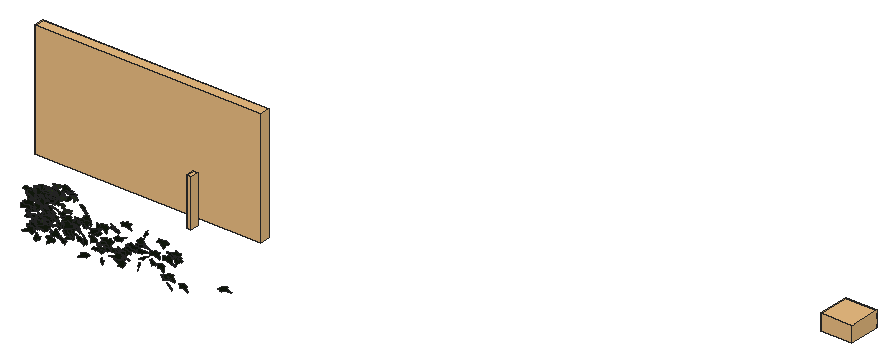
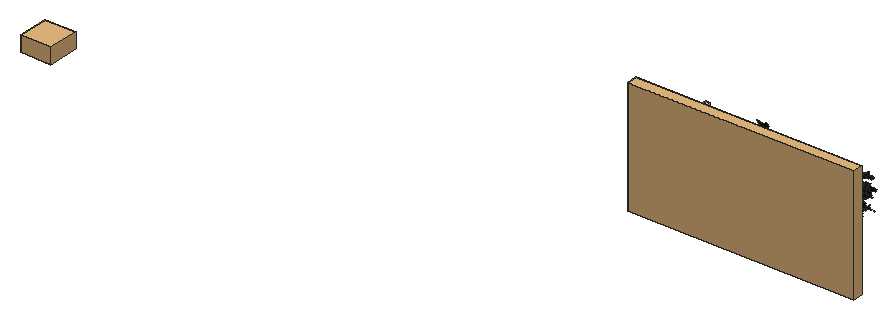
# SketchUp Ruby script. Lengths in millimetres.
U = 1.mm
M = Sketchup.active_model
def pt(a) = Geom::Point3d.new(a.map { |v| v * U })
def face(e, loops, mat)
  f = e.add_face(loops[0].map { |a| pt(a) })
  loops[1..].each { |l| e.add_face(l.map { |a| pt(a) }).erase! }
  f.material = f.back_material = mat if mat
  f
end
# faces: each face lists its corners as indices into pts; further lists are holes
def faces(e, pts, list, mat = nil) = list.each { |f| face(e, (f[0].is_a?(Array) ? f : [f]).map { |l| l.map { |i| pts[i] } }, mat) }
# xy, xz, yz: faces in a plane at the given z, y or x. An outline is a flat list of corners, or four numbers for a rectangle; further outlines are holes
def ring(l) = l.size == 4 ? [[l[0], l[1]], [l[2], l[1]], [l[2], l[3]], [l[0], l[3]]] : l.each_slice(2).to_a
def flat(e, list, mat, &to3) = list.each { |f| face(e, (f[0].is_a?(Array) ? f : [f]).map { |l| ring(l).map { |u, v| to3.(u, v) } }, mat) }
def xy(e, z, list, mat = nil) = flat(e, list, mat) { |x, y| [x, y, z] }
def xz(e, y, list, mat = nil) = flat(e, list, mat) { |x, z| [x, y, z] }
def yz(e, x, list, mat = nil) = flat(e, list, mat) { |y, z| [x, y, z] }
def lines(e, pts, list) = list.each { |a, b| e.add_line(pt(pts[a]), pt(pts[b])) }
# prism: a flat outline (further loops are holes) pulled along v
def prism(e, loops, v, mat = nil)
  f = face(e, loops, mat); d = Geom::Vector3d.new(v.map { |x| x * U })
  f.pushpull(f.normal.samedirection?(d) ? d.length : -d.length)
end
def box(e, o, s, mat = nil) = prism(e, [[o, [o[0] + s[0], o[1], o[2]], [o[0] + s[0], o[1] + s[1], o[2]], [o[0], o[1] + s[1], o[2]]]], [0, 0, s[2]], mat)
def at(x, y, z, deg = 0) = Geom::Transformation.translation(pt([x, y, z])) * Geom::Transformation.rotation(ORIGIN, Z_AXIS, deg.degrees)
def axes(o, x, y, z) = Geom::Transformation.new([*x, 0, *y, 0, *z, 0, *pt(o).to_a, 1])
def part(name) = M.definitions.add(name)
# library, detail: a bought-in or finely detailed component or shape, given as its bounding box
def library(name, o, s) = part(name).tap { |d| box(d.entities, o, s) }
def detail(e, o, s) = box(e.add_group.entities, o, s)
def put(e, d, t, mat = nil) = e.add_instance(d, t).tap { |i| i.material = mat if mat }
def group(e, t, mat = nil) = e.add_group.tap { |g| g.transformation = t; g.material = mat if mat }.entities
root = M.entities
M.materials.add("efeu1").color = [18, 25, 13]
M.materials.add("efeu2").color = [43, 57, 29]
c1 = part("ivyleaf_9")
p = [[39.1,54.8,31.7],[34.5,51.8,30.2],[-5.3,25.2,17.3],[-17.9,28.3,20.9],[-21.6,21.7,17],[-20.2,4.3,5.3],
  [-22.9,-0.3,2.5],[-17.1,-4,-0.6],[-2,-2.1,-1.2],[-0.7,-15.4,-10.1],[16.6,-22.3,-16.7],[21.1,-15.1,-12.5],
  [32.7,-10.7,-11],[46.1,-1.8,-6.6],[30.8,11.2,3.8]]
faces(c1.entities,p,[[0,1,2,3,4,5,6,7,8,9,10,11,12,13,14]],"efeu1")
c2 = part("ivyleaf_10")
p = [[0,12.8,-0.8],[-1.5,51.3,-10.9],[-4.9,51,-11.6],[-13.6,26.5,-7.3],[-13.2,15.9,-4.6],[-21.1,19.3,-7.2],
  [-29.5,16.3,-8.3],[-29.2,8.3,-6.2],[-19.7,-9.8,0.5],[-7.6,-13,4],[1,-12.2,5.8],[-0.4,51.1,-11.1],
  [-1.5,51.1,-10.9],[1,-12.4,5.9],[16.9,-12.4,3.5],[35.1,9.1,-5.1],[35,12.9,-6.1],[20.5,16.4,-4.9],
  [15.8,15,-3.8],[15.3,27.6,-7.1],[12.8,31.3,-7.8]]
faces(c2.entities,p,[[0,1,2,3,4,5,6,7,8,9,10],[11,12,0,13,14,15,16,17,18,19,20]],"efeu2")
c3 = library("EP Casement KUN43",[213.5,133.1,19],[2173.1,999.9,208])
c4 = library("Group\#28",[0,0,0],[80,165.5,939.4])
c5 = library("Dome Light",[-304.8,-304.8,0],[609.6,609.6,304.8])
put(root,c1,axes([6733.7,505.3,4189.8],[-1.97206,-0.38841,-0.73525],[1.30856,0.26051,-1.10658],[0.89009,-1.24354,-0.00217]))
put(root,c2,axes([6742.5,692.9,4090.2],[-0.42739,-1.00494,0.74621],[0.2241,-0.77172,-1.00386],[2.37165,-0.10818,0.22933]))
put(root,c1,axes([6750.8,560.4,4058.1],[-1.36315,-0.97569,0.43488],[-0.38923,-0.38865,-1.20881],[1.99542,-0.74234,0.06129]))
put(root,c1,axes([6769.7,727,3738.3],[-1.43892,0.87844,-0.32614],[0.36435,-0.26542,-1.15868],[-1.74575,-0.77945,0.02699]))
put(root,c1,axes([6714.2,723.1,3575],[1.48534,-1.0117,0.33632],[0.38922,-0.26701,-1.27774],[1.99139,0.80679,-0.00112]))
put(root,c2,axes([6728,785.8,3815.3],[-1.66169,0.14815,-0.79472],[1.4568,-0.22477,-0.88284],[-0.4949,-1.15904,0.06963]))
put(root,c1,axes([6804.6,567.8,3846.7],[-0.96065,-0.53842,-1.19678],[-1.48821,-0.90637,0.73756],[-2.00581,0.93035,0.02594]))
put(root,c1,axes([6728,434.6,3934.4],[-0.7611,-0.71245,-1.16865],[1.13859,1.00407,-0.81683],[2.34289,-0.71939,0.01732]))
put(root,c1,axes([6715.4,736.6,3954.7],[2.03916,-0.38469,0.4275],[0.82077,-0.06057,-1.13537],[0.72411,1.15198,0.08306]))
put(root,c1,axes([6813.1,672.8,4116.9],[-1.00585,0.07431,-1.11335],[-2.11438,0.07989,0.5327],[0.19813,1.22983,0.03267]))
put(root,c2,axes([6784.1,639.6,4142.7],[-1.42747,0.83417,0.54696],[-0.77928,0.36656,-1.12051],[-1.73114,-0.85286,0.05339]))
put(root,c2,axes([6790.2,696.8,4118.3],[-1.89408,-0.76625,0.11351],[-0.14108,-0.08974,-1.25576],[1.46748,-0.99763,0.02578]))
put(root,c1,axes([6756.8,719.5,4034.8],[2.01334,-0.51386,-0.29762],[-0.49832,0.1421,-1.176],[1.01438,1.08971,0.01301]))
put(root,c1,axes([6756.4,749.5,3900.3],[1.05397,-1.04409,-0.22406],[-0.00261,0.2517,-1.17629],[2.03236,0.54179,0.11468]))
put(root,c1,axes([6737.4,491.8,3912],[0.32662,0.07654,-1.2715],[2.28774,0.41479,0.18721],[0.80217,-1.21413,-0.0162]))
put(root,c1,axes([6792.2,489.3,3563.2],[-0.1903,-0.05994,1.23584],[-1.22329,-1.05693,-0.10327],[2.01215,-0.64823,0.0541]))
put(root,c1,axes([6799,1025.8,3947.2],[-2.15159,-0.31041,-0.27835],[0.51397,0.0677,-1.17234],[0.60455,-1.16231,0.00605]))
put(root,c1,axes([6772.1,713.1,3843.7],[0.50384,-0.96776,-0.66949],[-0.01953,0.6843,-0.99322],[2.23953,0.22369,0.14196]))
put(root,c2,axes([6790.8,1031.5,3963.5],[-0.24041,1.19336,0.10403],[-0.0249,0.10323,-1.20002],[-2.27967,-0.12698,0.00214]))
put(root,c1,axes([6823,698.8,4075.3],[-1.39529,0.82699,-0.51134],[0.20099,-0.56889,-1.07148],[-1.83955,-0.68943,0.27077]))
put(root,c1,axes([6752.3,567,3969.2],[2.47662,-0.53558,0.38455],[0.6748,-0.14889,-1.4072],[1.05797,1.34873,-0.00264]))
put(root,c1,axes([6837.6,690.2,3618.9],[-2.07239,0.63883,0.13083],[-0.21091,0.06965,-1.26245],[-1.223,-1.09451,-0.00398]))
put(root,c2,axes([6793.9,733,3896.5],[0.52832,1.16649,0.12122],[0.02339,0.12167,-1.19896],[-2.2319,0.2774,0.01613]))
put(root,c1,axes([6775.9,719.9,3887.7],[1.53097,-0.88299,-0.17271],[-0.05291,0.20718,-1.18866],[1.71154,0.79624,0.11775]))
put(root,c1,axes([6755.5,542.7,4016.6],[0.50999,-0.31854,1.34313],[2.15898,-0.72877,-0.39916],[1.49692,1.15961,0.1181]))
put(root,c2,axes([6813.3,714.9,4116],[-1.37441,-1.01441,-0.07105],[0.22611,0.00239,-1.24156],[1.9221,-0.72564,0.09525]))
put(root,c2,axes([6808.3,739.8,3919],[-1.58156,-0.78669,-0.40615],[0.63936,0.2352,-1.1429],[1.55898,-0.89454,0.05668]))
put(root,c1,axes([6798.4,558.1,3571.8],[0.06086,-1.35517,-0.01433],[-0.00283,0.0143,-1.35555],[2.5793,0.03199,-0.00115]))
put(root,c1,axes([6797.1,409.5,3845.6],[1.44273,-1.11985,-0.5426],[-0.55954,0.45619,-1.35225],[2.30126,0.81299,0.01138]))
put(root,c2,axes([6830.4,840.6,3789.3],[-0.65602,-0.48608,1.04457],[0.21568,-1.09933,-0.47417],[2.18209,-0.03748,0.3609]))
put(root,c1,axes([6800.6,719.1,4078.6],[2.24447,-0.37647,-0.00417],[0.00777,0.02649,-1.23766],[0.7165,1.17902,0.02648]))
put(root,c1,axes([6836.3,417.5,3759.7],[1.89186,0.23425,1.01453],[-1.88353,-0.22337,1.02125],[0.61588,-1.40268,0.0068]))
put(root,c1,axes([6816.6,854,3756.7],[2.20371,0.32052,-0.06017],[-0.12799,0.01752,-1.20094],[-0.60733,1.15933,0.03478]))
put(root,c2,axes([6843.4,695.6,4151.9],[2.29913,-0.07189,-0.3706],[-0.62789,0.40288,-1.15356],[0.34921,1.19765,0.3658]))
put(root,c1,axes([6888,409,3546.2],[-2.47976,0.04477,0.61869],[-1.17597,0.03319,-1.30367],[-0.10405,-1.44199,-0.01079]))
put(root,c1,axes([6811.9,666.4,3697.7],[1.88433,-0.7996,-0.19163],[-0.26525,0.1324,-1.27256],[1.54225,0.99973,0.01527]))
put(root,c1,axes([6808.4,743.7,3820.3],[1.57624,-0.88045,0.09053],[0.18769,-0.03142,-1.20772],[1.67402,0.83255,0.05017]))
put(root,c1,axes([6794.3,762.3,3587.1],[1.36344,0.83411,-0.95031],[0.9909,0.80075,1.09534],[2.19302,-0.8804,0.0959]))
put(root,c1,axes([6826.3,467.5,4181.3],[-0.07981,-1.30498,-0.14788],[0.00378,0.1479,-1.30565],[2.49953,-0.04189,-0.00275]))
put(root,c1,axes([6869.5,730.9,3998.6],[0.00718,1.13496,-0.42983],[-0.36779,-0.42379,-1.1207],[-2.28031,0.07193,0.1794]))
put(root,c1,axes([6819.3,676.5,3842.2],[0.83503,-1.10688,0.21512],[0.18598,-0.19263,-1.1905],[2.13795,0.44908,0.01955]))
put(root,c1,axes([6849.4,998.2,3992.2],[1.99516,0.46198,-0.49603],[-0.83353,-0.23562,-1.14504],[-0.98465,1.13556,-0.03579]))
put(root,c1,axes([6839.9,701,4152.4],[-0.52752,-0.01712,-1.20854],[2.02074,-0.5959,-0.23507],[-1.09913,-1.08733,0.14786]))
put(root,c1,axes([6886.5,715.9,3700.5],[-0.74386,1.1112,-0.27155],[0.11378,-0.26672,-1.17752],[-2.17409,-0.39415,0.03129]))
put(root,c1,axes([6840.3,491.3,3724.5],[0.71413,-1.33961,-0.14677],[-0.06772,0.14245,-1.39116],[2.56391,0.37689,0.00414]))
put(root,c2,axes([6847,487.1,3759.4],[2.10945,0.46078,0.33823],[0.61517,0.10335,-1.20002],[-0.8972,1.15421,-0.02758]))
put(root,c1,axes([6873.8,618,4140.6],[-0.73463,-0.92053,0.87757],[-0.71257,-0.79421,-0.99777],[2.31325,-0.53698,-0.02866]))
put(root,c2,axes([6849.5,532.3,4073.6],[1.62485,-0.55107,0.72463],[1.11722,-0.42607,-1.01564],[1.3243,1.03559,-0.03226]))
put(root,c1,axes([6852.7,672.5,3957.8],[0.07165,-1.19958,-0.181],[0.07963,0.18226,-1.19925],[2.30752,0.03096,0.047]))
put(root,c2,axes([6884.6,1030,4061.3],[-2.30409,-0.06486,-0.03905],[0.08643,-0.12161,-1.20604],[0.11528,-1.20515,0.1238]))
put(root,c2,axes([6880.7,696.6,3609],[2.23824,-0.24952,-0.06652],[-0.12849,0.00227,-1.20216],[0.47438,1.17792,-0.01177]))
put(root,c1,axes([6907.8,695.7,4175.9],[-2.11493,-0.55593,0.28897],[-0.48531,-0.13614,-1.24253],[1.08922,-1.14011,0.00747]))
put(root,c1,axes([6837.4,701.2,4134.1],[0.70044,0.018,-1.29043],[2.41406,0.24243,0.36514],[0.45297,-1.31981,0.04947]))
put(root,c1,axes([6856.4,336.8,4076.2],[-0.57288,-0.37439,-1.43914],[1.7138,1.12261,-0.48039],[2.25223,-0.94946,-0.00052]))
put(root,c1,axes([6855.9,657.6,3531.1],[0.65849,0.21406,-1.23678],[0.97642,1.14672,0.34199],[2.18017,-0.57823,0.22038]))
put(root,c1,axes([6844.6,459.6,3614.6],[0.90183,-0.1849,-1.36218],[2.61397,0.12404,0.46094],[0.1096,-1.4369,0.21508]))
put(root,c2,axes([6906.7,729.7,4127.2],[0.4479,-1.16667,0.30849],[0.03686,-0.3106,-1.18946],[2.29642,0.23254,-0.04108]))
put(root,c2,axes([6913.9,734.2,4013.4],[1.61593,0.7393,-0.47951],[-0.67757,-0.32132,-1.12579],[-1.53411,0.92065,-0.00786]))
put(root,c2,axes([6911.6,719.6,3907.7],[-1.48928,0.9289,0.0317],[-0.05758,0.01596,-1.2145],[-1.76797,-0.78299,0.01285]))
put(root,c1,axes([6889.1,718.4,4140.7],[0.60189,-1.14285,-0.3785],[-0.02657,0.38784,-1.1827],[2.29111,0.30473,0.08572]))
put(root,c2,axes([6909.1,733.3,3884],[-0.04898,1.19278,-0.26648],[0.04079,-0.26606,-1.19296],[-2.32571,-0.02979,-0.01531]))
put(root,c2,axes([6898.4,721.9,3755.7],[0.05212,-0.62171,1.04311],[1.2466,-0.87102,-0.53633],[1.94609,0.5746,0.31562]))
put(root,c2,axes([6906.4,734.3,4044.3],[-1.2808,0.61483,-0.8062],[0.95767,-0.63751,-0.90622],[-1.67521,-0.83452,0.09833]))
put(root,c2,axes([6930.8,1065.6,3927],[0.02848,1.05734,-0.66458],[-0.17,-0.66202,-1.05528],[-2.37073,0.06017,0.06769]))
put(root,c1,axes([6915.8,711.9,3780.8],[1.21349,-0.84412,-0.67888],[-0.43839,0.66408,-1.04206],[2.01447,0.653,0.18217]))
put(root,c2,axes([6949.1,751.6,4006],[-0.73935,-1.14887,0.01493],[-0.03681,-0.00922,-1.21267],[2.1864,-0.38865,-0.01536]))
put(root,c1,axes([6923.4,557.1,3560],[0.33599,-0.86219,-0.98097],[-0.24565,0.97353,-0.87888],[2.47344,0.21381,0.04596]))
put(root,c2,axes([6935.1,721.7,4152],[1.73745,-0.8154,-0.0325],[0.45971,0.31658,-1.15792],[1.48351,0.85688,0.39687]))
put(root,c1,axes([6953.2,480,3969.2],[-1.33397,-1.03439,0.17022],[-0.19841,-0.13497,-1.24945],[1.98524,-0.70854,-0.01049]))
put(root,c1,axes([6932.7,708.4,4159.6],[-0.14552,-1.24239,-0.11518],[0.09615,0.11222,-1.24398],[2.37271,-0.08074,0.04335]))
put(root,c1,axes([6958.5,772.7,3942.3],[0.48064,0.62101,1.0079],[0.43262,0.98596,-0.66445],[-2.21118,0.32789,0.08908]))
put(root,c2,axes([6949.9,731.2,3994],[1.57349,-0.84888,0.3221],[0.55061,-0.16662,-1.18171],[1.63792,0.87151,0.08781]))
put(root,c1,axes([6946.2,728.4,4155.8],[0.65249,-1.15534,-0.25454],[-0.012,0.26323,-1.20325],[2.25154,0.33622,0.06735]))
put(root,c1,axes([6979.9,659,4134.6],[-2.01163,-0.60589,-0.18367],[0.32683,0.06967,-1.21806],[1.15977,-1.07055,0.02468]))
put(root,c1,axes([6973.7,507.1,3660.3],[-1.36168,-1.09559,0.17966],[-0.15842,-0.1602,-1.30839],[2.10702,-0.72008,0.01773]))
put(root,c1,axes([6953.4,702.4,4106.9],[2.18676,0.41498,0.05925],[0.10949,0.01512,-1.22162],[-0.79025,1.15042,-0.00532]))
put(root,c1,axes([6962.5,698.1,3755.5],[-1.56977,-0.6044,-0.80135],[1.27379,0.44178,-1.02208],[1.4236,-1.06174,0.03089]))
put(root,c2,axes([6974.6,669.9,4078],[-1.62611,-0.7552,-0.45913],[0.69655,0.27895,-1.13991],[1.53108,-0.92898,0.03096]))
put(root,c2,axes([6988,1066.2,3890.5],[1.34458,-1.01724,-0.1451],[-0.1878,0.10811,-1.23835],[1.94656,0.71308,-0.01925]))
put(root,c1,axes([7002.1,621.6,4120.7],[-1.79767,-0.75306,-0.43916],[0.69625,0.24534,-1.20752],[1.50598,-1.01235,0.03404]))
put(root,c1,axes([7022.6,648.4,3798.8],[-1.35814,-0.84052,0.81421],[-0.99976,-0.62208,-1.10259],[1.99014,-0.8861,0.00175]))
put(root,c1,axes([7039.2,1112.4,3996.3],[-2.34104,0.22373,0.09712],[-0.17656,0.03263,-1.25014],[-0.42931,-1.23345,-0.01545]))
put(root,c1,axes([6987.7,645.7,3741],[-0.66906,-1.20696,-0.64325],[0.56479,0.58102,-1.25238],[2.54094,-0.44695,0.109]))
put(root,c1,axes([6969.6,622,3652.3],[2.31496,-0.61794,0.36407],[0.62651,-0.15581,-1.36428],[1.21273,1.26007,0.00984]))
put(root,c1,axes([7085.7,682.3,4044.8],[-1.97076,-0.05838,0.68681],[-1.27206,-0.21794,-1.02623],[0.32067,-1.2233,0.15005]))
put(root,c2,axes([7029.1,691.2,4156.3],[-1.96383,-0.37718,-0.54841],[1.18173,-0.18105,-1.04376],[0.45629,-1.15443,0.34287]))
put(root,c2,axes([7046.5,730.1,4088.5],[0.48812,0.92168,-0.76849],[-0.48948,-0.72537,-0.95579],[-2.23083,0.36083,0.04156]))
put(root,c1,axes([7035.5,725,4052.4],[0.05748,-1.23454,0.00848],[0.00043,-0.00847,-1.23491],[2.34963,0.0302,0.00002]))
put(root,c2,axes([7052.2,724.2,3974.4],[-0.02369,0.99855,-0.72682],[-0.1739,-0.72561,-0.99533],[-2.34413,0.04374,0.08118]))
put(root,c2,axes([7017,728,3947.6],[1.30725,-0.12482,-1.01492],[1.93595,-0.04157,0.69353],[-0.19894,-1.22479,0.07989]))
put(root,c1,axes([7026,607.2,4102.4],[1.57163,-1.15992,-0.03923],[-0.04323,0.03198,-1.42384],[2.2084,0.82609,0.00004]))
put(root,c1,axes([7081.1,375.8,3901.6],[-1.1883,0.95631,-0.70967],[0.69847,-0.60778,-1.14189],[-2.15614,-0.72393,0.02121]))
put(root,c2,axes([7058.8,1059.5,4009.6],[-2.22684,0.09928,-0.46292],[0.87686,-0.04536,-1.17424],[-0.20744,-1.25748,0.00581]))
put(root,c1,axes([7087.3,1016.5,4093.4],[-2.14063,-0.4794,-0.04315],[0.0744,0.01833,-1.22266],[0.91305,-1.12543,-0.00153]))
put(root,c1,axes([7051.3,721.1,3861.7],[2.31616,-0.1043,-0.08314],[-0.139,0.11741,-1.21644],[0.21241,1.21416,0.11049]))
put(root,c1,axes([7051.1,642.4,3652.3],[1.04338,1.03089,-0.57968],[0.48578,0.52075,1.16748],[2.19786,-0.60449,0.01715]))
put(root,c1,axes([7120.7,664,4098.7],[0.63611,1.02024,-0.62057],[-1.26091,-0.37772,-0.97781],[-1.89085,0.5951,0.44328]))
put(root,c1,axes([7070.8,563.7,3632.6],[0.13589,0.52873,-1.29242],[0.25894,1.28531,0.53334],[2.64495,-0.153,0.01419]))
put(root,c1,axes([7113.5,1023.1,4033.6],[0.97559,1.13395,-0.20258],[-0.53899,-0.09087,-1.22523],[-2.12502,0.54364,0.21776]))
put(root,c1,axes([7103.5,720.7,4102],[-1.26938,-1.02849,-0.18823],[0.25111,0.13869,-1.22533],[1.97403,-0.679,0.03483]))
put(root,c1,axes([7140.4,230.4,3555],[-2.08077,0.60329,-0.55811],[-0.93825,0.26175,1.24868],[1.2515,1.19928,0.00822]))
put(root,c2,axes([7104.7,721.8,4007.5],[1.58392,-0.89057,0.22858],[0.45153,-0.08987,-1.21393],[1.69061,0.85837,0.11006]))
put(root,c1,axes([7070.2,728.7,4115.4],[1.53703,-0.6856,0.62738],[0.95585,-0.37735,-1.05889],[1.48817,0.95049,0.03215]))
put(root,c1,axes([7117.7,722,4131.5],[1.36463,1.00502,-0.03351],[-0.03875,-0.02664,-1.23458],[-1.91343,0.7173,0.0011]))
put(root,c1,axes([7089.7,572.9,3681.8],[0.54682,-0.78886,0.90976],[0.60756,-0.85193,-0.83953],[2.20972,0.42945,0.0057]))
put(root,c1,axes([7073,558.2,3665.5],[0.90847,-0.33274,1.16148],[2.00426,-0.49756,-0.57534],[1.12712,1.15296,0.08691]))
put(root,c1,axes([7094.9,727.2,4106.8],[1.53579,-0.89437,0.2562],[0.28015,-0.21213,-1.20417],[1.74832,0.81964,-0.0321]))
put(root,c1,axes([7187.5,495.4,3910.3],[-0.39153,0.1631,1.47402],[-2.62627,0.52409,-0.25058],[-1.03395,-1.39298,0.07831]))
put(root,c1,axes([7154,717.7,4036.1],[0.17498,1.23358,-0.1325],[-0.01355,-0.13234,-1.237],[-2.36122,0.09217,-0.00272]))
put(root,c2,axes([7137.7,601.5,3868.9],[-1.87919,0.68872,-0.31477],[0.51634,-0.16117,-1.20365],[-1.34552,-1.02374,-0.02227]))
put(root,c1,axes([7110.1,580.3,3554.6],[1.31225,-0.85409,0.56382],[0.65995,-0.44466,-1.09764],[1.83254,0.77173,-0.00845]))
put(root,c1,axes([7180.7,507.4,4124.6],[-0.17315,0.72057,-1.21261],[0.02314,-1.21469,-0.72271],[-2.68446,-0.05695,0.07198]))
put(root,c1,axes([7213.8,367.1,3702.7],[-0.85017,-0.19552,1.39444],[-2.43779,-0.55116,-0.48761],[1.113,-1.35655,-0.00286]))
put(root,c1,axes([7212.4,605.3,3772.1],[-1.07625,-0.94835,-0.6007],[-0.58177,-0.51711,1.10415],[-2.05578,0.64282,0.00202]))
put(root,c2,axes([7191.3,680.8,4129.4],[-2.28562,-0.29196,0.04887],[-0.09504,-0.00147,-1.23587],[0.55532,-1.20193,-0.01036]))
put(root,c1,axes([7181.3,481.1,4134.1],[1.7699,1.12425,-0.03206],[-0.03902,-0.02464,-1.45902],[-2.14018,0.93018,0.00009]))
put(root,c1,axes([7179,720.3,4171],[-0.10468,-1.14343,0.47918],[-0.10042,-0.47706,-1.14442],[2.3574,-0.0711,-0.02747]))
put(root,c1,axes([7174,481.3,3891.6],[1.61266,-0.83471,0.6193],[0.8284,-0.4406,-1.1894],[1.79629,0.95257,-0.00747]))
put(root,c1,axes([7184.1,479.2,4012.7],[-0.41509,0.04436,-1.40532],[2.65623,-0.16546,-0.22182],[-0.32419,-1.41249,-0.01815]))
put(root,c1,axes([7243.1,642.2,3638.9],[-0.77727,-1.08907,0.62257],[0.52301,0.56116,1.16191],[-2.32949,0.48937,0.05314]))
put(root,c1,axes([7249.7,611.9,4061.3],[-0.54356,-0.4246,1.23886],[-1.02823,-1.11685,-0.50733],[2.27045,-0.60744,0.06683]))
put(root,c2,axes([7249.5,712.7,4094.2],[0.81385,-1.12991,-0.3278],[-0.07216,0.33537,-1.20545],[2.23795,0.42172,0.08034]))
put(root,c1,axes([7211.6,763.1,3730.3],[1.90806,0.41943,0.63751],[1.12288,0.24153,-1.08674],[-0.92112,1.16327,-0.00422]))
put(root,c1,axes([7289.5,813.6,4044.2],[-0.57252,0.90709,0.7921],[-0.97036,0.64372,-0.9308],[-2.0764,-0.55094,0.21659]))
put(root,c1,axes([7282.6,911.4,4092.9],[0.79032,1.03316,-0.55982],[-0.91715,-0.39179,-1.08052],[-2.0397,0.57648,0.26895]))
put(root,c1,axes([7303.9,468.9,3559.2],[-2.4151,0.13569,0.56556],[1.0692,-0.06543,1.27619],[0.28655,1.38776,0.00487]))
put(root,c2,axes([7322.5,656.3,4153.2],[-1.13341,-0.97457,0.53729],[-0.39121,-0.50257,-1.13942],[2.08155,-0.6251,0.07841]))
put(root,c1,axes([7362.3,598.9,3906.4],[-1.16946,1.00994,0.46058],[-0.42129,0.40437,-1.18202],[-2.07013,-0.65283,-0.01964]))
put(root,c1,axes([7353.6,306.9,3596.8],[-1.67937,-1.01863,0.44685],[-0.57583,-0.32907,-1.34761],[2.03717,-0.93274,-0.01255]))
put(root,c2,axes([7326.6,601.7,4050.7],[-1.01637,0.43125,-1.04757],[1.14623,-0.87283,-0.66634],[-1.82613,-0.78788,0.1648]))
put(root,c2,axes([7402.9,820.3,4111.9],[2.1993,-0.47439,0.09499],[0.17572,-0.02523,-1.24911],[0.90386,1.1592,0.01169]))
put(root,c1,axes([7412.3,720.1,3651.5],[-0.00163,-0.1969,-1.27513],[0.63351,1.23193,-0.19046],[2.37246,-0.32909,0.04998]))
put(root,c1,axes([7414.8,485.8,3499],[-0.13408,0.03062,1.32356],[1.01243,-1.21308,0.05638],[2.30733,0.53406,0.05217]))
put(root,c2,axes([7462.6,561.7,4020.6],[-2.04643,-0.33062,-0.59086],[1.06948,0.18279,-1.12491],[0.71882,-1.21321,-0.00847]))
put(root,c1,axes([7478.3,797.9,3577.2],[1.99164,-0.84996,-0.22331],[-0.31962,0.14743,-1.34813],[1.64172,1.05982,0.00844]))
put(root,c1,axes([7497.6,287.8,3868.6],[-0.13678,0.09407,1.37404],[0.38548,-1.36023,0.10372],[2.5927,0.2072,0.05707]))
put(root,c1,axes([7543.8,579.4,3634.8],[1.49755,0.89633,-0.4783],[-0.65805,-0.3326,-1.19212],[-1.81815,0.85866,0.03751]))
put(root,c3,axes([4878.1,2667.2,3134.8],[2.04542,0,0],[0,0,2.2766],[0,-1,0]))
put(root,c1,axes([7577.3,493,3940.9],[-1.75451,-0.63282,0.88161],[-1.43155,-0.46123,-1.1176],[1.48878,-1.18926,-0.03568]))
put(root,c1,axes([7585.3,677,3859.3],[0.78307,0.31446,-1.17085],[-2.1999,-0.27112,-0.47901],[-0.69582,1.21106,0.19678]))
put(root,c1,axes([7593.8,485.7,3653.3],[-1.79234,-0.80924,0.59251],[-0.82026,-0.40738,-1.24142],[1.72361,-1.03538,0.02535]))
put(root,c1,axes([7600.5,306.3,3925.5],[-1.50899,1.04868,-0.4294],[0.50097,-0.3393,-1.31467],[-2.0977,-0.8354,-0.00508]))
put(root,c1,axes([7565.3,419.1,3761.6],[0.2135,-0.93482,-1.10907],[0.0772,1.11397,-0.93485],[2.7595,0.04116,0.11196]))
put(root,c1,axes([7608,635.8,3826.6],[0.51826,-1.09893,-0.7821],[0.39183,-0.75467,1.13207],[-2.53701,-0.34104,0.01508]))
put(root,c1,axes([7617.8,653.4,3715.5],[1.1447,-0.31189,-1.17913],[-2.04608,0.48537,-0.67677],[1.09635,1.23147,-0.03189]))
put(root,c1,axes([7593.5,482.1,3711.1],[-1.08876,1.30133,0.53014],[0.35401,-0.49722,1.42125],[2.65079,0.6009,0.02794]))
put(root,c1,axes([7629.1,293.5,3840.6],[1.71166,-1.00736,-0.6554],[-0.73111,0.53469,-1.34897],[2.16728,0.97596,0.06256]))
put(root,c1,axes([7600.5,328,3922.3],[1.51928,-0.19444,1.12405],[2.06529,-0.29358,-0.82145],[0.66942,1.34705,-0.01678]))
put(root,c1,axes([7649.5,711.7,4038.2],[1.84471,-0.4397,-0.7493],[-1.15215,0.46339,-1.05502],[1.18597,1.13411,0.14057]))
put(root,c1,axes([7702.6,810.3,3784.5],[0.55296,-0.04804,-1.27083],[-2.40532,0.1342,-0.29402],[0.26942,1.29669,-0.01665]))
put(root,c1,axes([7680.9,609.2,3907.1],[0.78043,0.37396,1.25976],[1.26205,1.08044,-0.53658],[-2.1592,0.76668,0.1417]))
put(root,c1,axes([7665.6,664.4,4121.6],[1.22921,-1.21892,0.28644],[0.29112,-0.24308,-1.3793],[2.36519,0.6634,0.02091]))
put(root,c1,axes([7742,261.3,4008.8],[-2.59889,-0.27359,-0.15204],[0.28466,0.02743,-1.39267],[0.52329,-1.3737,0.00248]))
put(root,c1,axes([7716.1,564.1,3913.6],[2.38658,0.36144,0.45038],[0.82145,0.12872,-1.30503],[-0.73018,1.32618,0.00392]))
put(root,c1,axes([7758.7,474.1,3679.1],[-0.36227,0.0059,-1.33006],[2.52747,0.07558,-0.18972],[0.14081,-1.34148,-0.01654]))
put(root,c1,axes([7816,544.2,3979.2],[-1.2072,-0.83386,-0.81317],[1.0873,0.58415,-1.04465],[1.93171,-0.84991,0.07982]))
put(root,c1,axes([7871.5,493.9,4086.5],[0.63463,-0.77229,-1.07963],[-0.46015,1.05921,-0.83236],[2.48407,0.39352,0.12164]))
put(root,c1,axes([7905.3,392.6,4007.9],[1.7609,-0.20574,-0.94708],[-1.75788,0.20937,-0.94783],[0.55864,1.30735,0.00275]))
put(root,c1,axes([7895.9,460.4,3691.6],[0.25193,-0.12922,-1.4706],[1.79597,-1.12806,0.18406],[-2.16067,-0.95272,-0.01848]))
put(root,c1,axes([8012,624.3,3770.3],[-0.28345,0.16182,1.37776],[-2.40434,0.55665,-0.20194],[-1.09074,-1.26908,0.0871]))
put(root,c1,axes([7997.5,548.8,3723],[-1.02769,-1.0524,0.877],[-0.47994,-0.8502,-1.17551],[2.56266,-0.58126,0.13154]))
put(root,c1,axes([8039.5,528.2,3898.4],[0.09766,0.73717,-1.19645],[-0.13111,-1.19449,-0.73891],[-2.67139,0.08557,-0.00747]))
put(root,c1,axes([8011.3,747.8,3570.8],[-0.06096,-0.54579,-1.27663],[0.16308,1.27376,-0.54671],[2.63738,-0.09138,0.0043]))
put(root,c1,axes([8060.6,750.9,3557.2],[-0.06648,0.08559,1.33642],[-0.22756,1.33134,-0.08839],[-2.53851,-0.12158,-0.02708]))
put(root,c1,axes([8067.6,252.4,3598.3],[-0.24741,0.2299,-1.40122],[-0.35988,-1.39735,-0.21172],[-2.67839,0.16652,0.15789]))
put(root,c1,axes([8072.4,450.6,3898.4],[1.03033,0.33338,1.21324],[-2.20951,-0.37685,0.62159],[0.92321,-1.27398,0.13362]))
put(root,c1,axes([8103.1,565.2,3921.2],[-2.03794,0.40282,-0.79971],[-1.43141,0.27192,1.14403],[0.92483,1.30851,0.00845]))
put(root,c1,axes([8048,489.4,3586.1],[1.93924,0.27131,0.93726],[1.7332,0.22214,-1.05434],[-0.66677,1.36651,-0.0147]))
put(root,c1,axes([8182.1,533.9,3574.1],[-1.46071,-1.13058,0.27093],[0.32499,0.21149,1.3663],[-2.18864,0.78596,0.02206]))
put(root,c1,axes([8204.5,779.7,3896.7],[0.68658,-1.11878,0.81087],[1.02726,-0.65736,-1.14711],[2.42076,0.59626,0.2568]))
put(root,c1,axes([8210.1,571.3,3623.4],[0.93593,-0.09644,-1.30697],[2.33656,0.5223,0.4234],[0.87263,-1.29507,0.26808]))
put(root,c1,axes([8257.6,410.5,3458.6],[-0.01797,0.42488,1.40918],[0.05801,-1.40885,0.42499],[2.80061,0.03191,0.00024]))
put(root,c1,axes([8311.9,796.6,3450.1],[-2.45453,-0.24558,0.32847],[0.61305,0.06434,1.31286],[-0.48314,1.3293,-0.00287]))
put(root,c1,axes([8297.3,430.9,4100.6],[-0.39597,-1.37478,-0.41183],[0.18726,0.40149,-1.38998],[2.72493,-0.22737,0.03568]))
put(root,c1,axes([8300.9,507.5,3747.3],[0.41907,-1.24411,-0.66524],[-0.05168,0.66943,-1.26094],[2.68454,0.2071,0.07957]))
put(root,c1,axes([8377.1,391.5,3879.4],[-2.74724,0.02843,0.02136],[-0.04073,-0.00196,-1.44376],[-0.05404,-1.44364,0.00238]))
put(root,c1,axes([8458,513.4,3697.1],[-0.86353,-1.04339,-0.84297],[0.72006,0.75421,-1.13717],[2.44924,-0.58961,0.03711]))
put(root,c1,axes([8444.9,468.7,4069.1],[2.44077,-0.27246,-0.62526],[1.2025,-0.02687,1.30765],[-0.48883,-1.42651,0.09479]))
put(root,c1,axes([8484.9,283.3,3985.7],[-1.74692,-0.68179,-0.92156],[1.35506,0.58619,-1.14283],[1.7099,-1.1611,-0.03584]))
put(root,c1,axes([8471.4,617,3590.3],[-0.42482,-0.10583,-1.41746],[2.70167,-0.09002,-0.21682],[-0.13842,-1.4321,0.11838]))
put(root,c1,axes([8562.4,502.7,3670.1],[1.36929,0.01913,1.28158],[-2.43819,-0.03512,0.71972],[0.0761,-1.4693,-0.00052]))
put(root,c1,axes([8585.7,724,3605.5],[0.55755,1.03713,0.86974],[0.47779,0.8328,-1.07765],[-2.53137,0.38562,-0.01184]))
put(root,c1,axes([8617.4,593.3,3704.2],[-2.36299,-0.11695,-0.761],[1.44138,0.07449,-1.24708],[0.26385,-1.45434,-0.00268]))
put(root,c1,axes([8617.4,550.3,4203.4],[-0.96706,-0.56858,-1.23636],[1.45271,0.97351,-0.7614],[2.14417,-0.91601,-0.04176]))
put(root,c1,axes([8637.7,330.2,4024.1],[0.15794,-0.10046,1.48711],[2.74959,0.3717,-0.05551],[-0.69762,1.44229,0.11789]))
put(root,c1,axes([8762,222,3806.8],[-2.26398,0.33144,0.84646],[-1.54244,0.24472,-1.23478],[-0.78359,-1.43933,-0.01503]))
put(root,c1,axes([8689.2,356.4,3766.7],[1.4227,-0.95085,0.86477],[1.27683,-0.56463,-1.20077],[2.08646,0.99389,0.14516]))
put(root,c1,axes([8760.1,675.5,3817.9],[2.15164,-0.07307,0.83744],[1.59429,-0.01914,-1.13255],[0.13346,1.40679,0.02809]))
put(root,c1,axes([8855,186.6,3729.5],[-1.40804,-1.24347,-0.37199],[-0.25853,-0.35165,1.44562],[-2.45664,0.74971,0.06108]))
put(root,c1,axes([8870.9,373,3893.4],[1.6997,-0.46326,1.08855],[-1.86097,0.47866,1.00593],[-1.26734,-1.32416,-0.0172]))
put(root,c1,axes([8886.1,549.7,3581.3],[-1.16583,0.43554,-1.27982],[1.97587,-0.74842,-0.75161],[-1.64801,-1.20542,0.00424]))
put(root,c1,axes([8889.3,561.6,3995.5],[0.65472,-0.78362,-1.19815],[-0.49236,1.17795,-0.84468],[2.67987,0.40787,0.13753]))
put(root,c1,axes([8956.3,556.5,3714.7],[0.84935,1.40732,0.05684],[0.03158,0.05436,-1.47638],[-2.6804,0.44658,0.00062]))
put(root,c1,axes([9023.1,535.7,4176.1],[0.11906,-0.08833,-1.49007],[-1.76042,1.16823,-0.10808],[2.22969,0.92707,-0.00577]))
put(root,c1,axes([9032.1,175.2,4098.7],[0.0136,0.02042,1.50665],[2.18744,-0.97437,0.00775],[1.85444,1.14919,-0.0202]))
put(root,c1,axes([9084.7,644.4,3642.9],[-0.44137,-0.93222,1.02547],[-0.27261,-1.01804,-0.95786],[2.62346,-0.26262,0.07299]))
put(root,c1,axes([9069,304.7,3978.3],[0.8385,-0.06293,1.39339],[2.62384,-0.20217,-0.44504],[0.40296,1.44733,-0.00158]))
put(root,c1,axes([9161.6,362.7,4085.2],[1.895,-0.39264,-0.88837],[1.55617,-0.3478,1.07016],[-0.99768,-1.28827,-0.01816]))
put(root,c1,axes([9177.3,553.1,3892.6],[-0.89851,-0.72282,-1.14476],[1.17034,0.96561,-0.8633],[2.29556,-0.77522,-0.00794]))
put(root,c4,at(9222.2,1292.1,4008))
put(root,c1,axes([9260.8,852.6,3637.6],[2.30821,-0.60857,-0.66557],[-1.14176,0.28841,-1.35689],[1.28157,1.35303,-0.01013]))
put(root,c1,axes([9325.2,523.9,3727.7],[-1.1314,-0.21062,-1.29138],[2.43598,0.20086,-0.62196],[0.51698,-1.40738,0.10449]))
put(root,c1,axes([9348.1,660.5,3819.9],[-0.91489,-0.78955,-1.10573],[1.10364,0.94147,-0.92437],[2.3385,-0.75322,0.00366]))
put(root,c1,axes([9411.6,481.3,4197.1],[-2.00682,-0.71823,-0.7846],[1.28107,0.40489,-1.27526],[1.56754,-1.25041,0.03773]))
put(root,c1,axes([9448.6,505.9,3568.7],[1.38789,0.61538,-1.08606],[-1.79075,-0.55557,-0.94658],[-1.56118,1.18433,0.12027]))
put(root,c1,axes([9512.6,721.8,3870.2],[-1.57495,0.11429,1.17983],[-2.21437,0.19668,-0.83513],[-0.43115,-1.42762,-0.02061]))
put(root,c1,axes([9479.2,510.5,3605.2],[-0.07029,-0.92342,-1.19789],[0.89457,1.13191,-0.88705],[2.73605,-0.39381,0.25925]))
put(root,c1,axes([9571.1,437.2,4048.7],[1.4728,-0.70973,1.07232],[1.61817,-0.65651,-1.04811],[1.83605,1.14792,0.06356]))
put(root,c1,axes([9706.4,484.8,3995.9],[-1.39166,-1.31011,0.1541],[-0.1352,-0.13683,-1.50035],[2.50695,-0.73465,0.00463]))
put(root,c1,axes([9741.7,213.6,3638.3],[-0.10646,-0.49184,1.39855],[0.62539,-1.36885,-0.46825],[2.75134,0.29211,0.16055]))
put(root,c1,axes([9871.7,389.9,3621.5],[-1.03025,-0.09997,-1.35765],[2.52153,0.29708,-0.55014],[0.59541,-1.43108,-0.01936]))
put(root,c1,axes([10470.9,614.6,3678.7],[0.01531,-0.02791,-1.51187],[0.78083,1.45522,-0.02468],[2.76992,-0.41007,0.01532]))
put(root,c5,at(19194.1,5128.3,4046.1))
